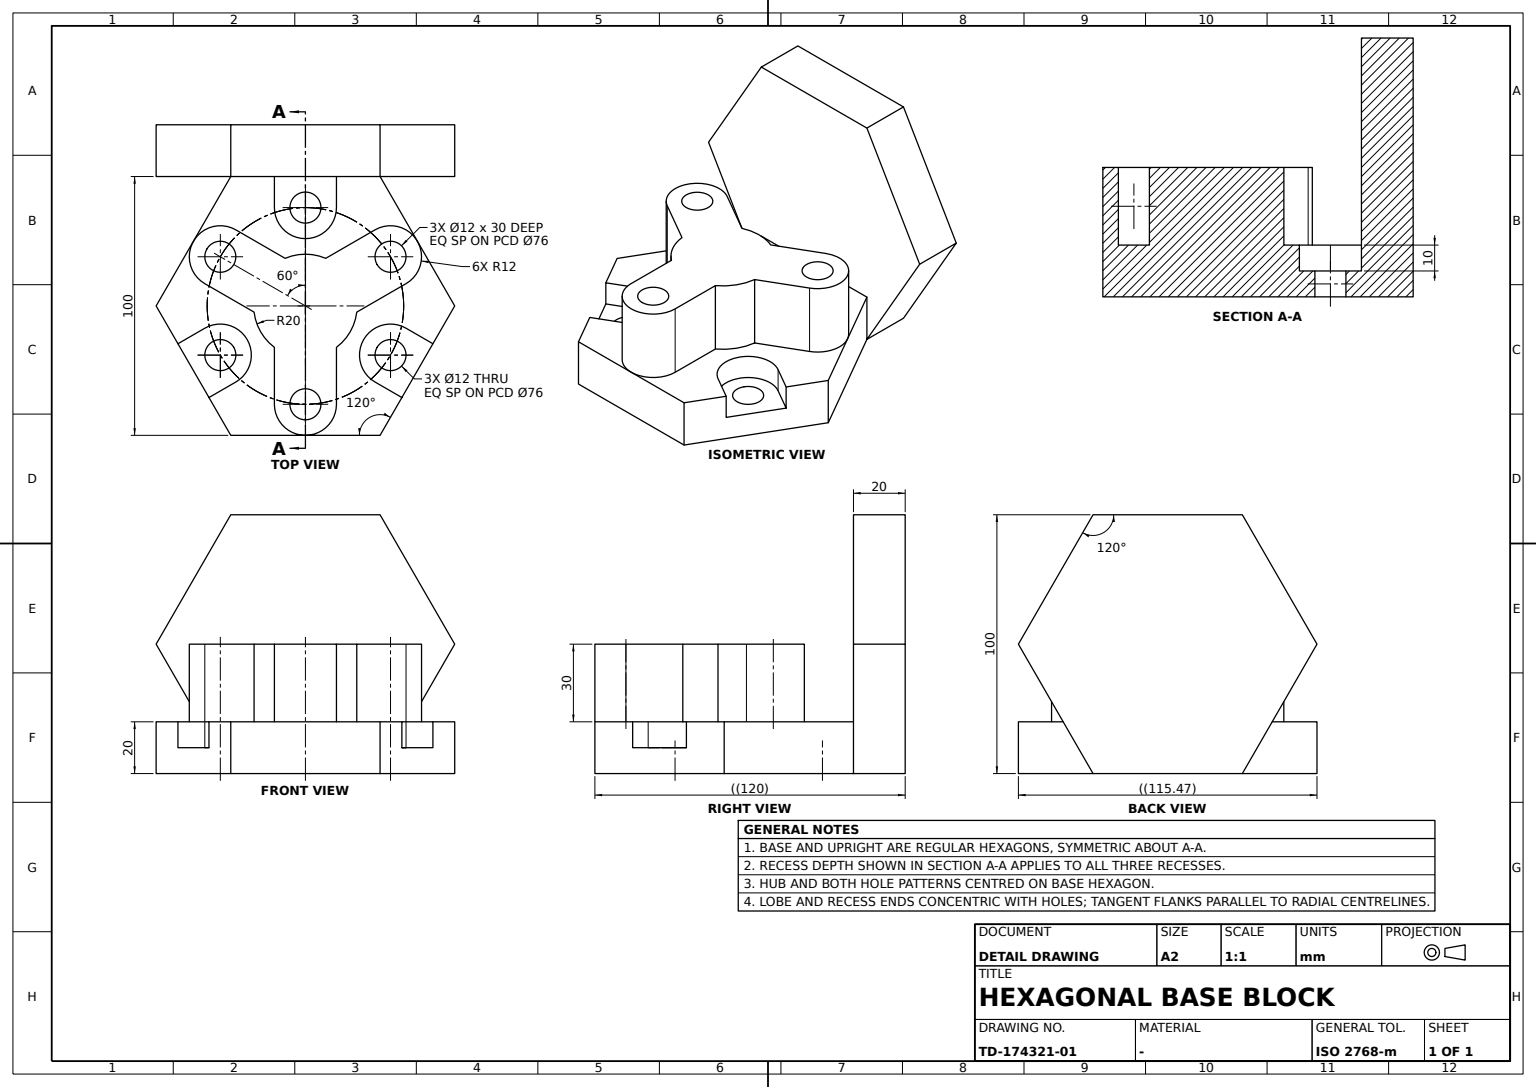
solid
v1 (-22,38.105118,20)
v2 (-22,38.105118,50)
e1 v1 v2 LINE
v3 (-13,32.908965,20)
e2 v3 v1 CIRCLE(AX(P(-19,32.908965,20),D(0,0,1),D(1,0,0)),6)
v4 (-13,32.908965,50)
e3 v4 v3 LINE
e4 v4 v2 CIRCLE(AX(P(-19,32.908965,50),D(0,0,1),D(1,0,0)),6)
face CYL(AX(P(-19,32.908965,35),D(0,0,-1),D(1,0,0)),6) rev [-e1 -e2 -e3 e4]
v5 (13.876084,29.787189,10)
v6 (16,27.712813,10)
e5 v5 v6 CIRCLE(AX(P(19,32.908965,10),D(0,0,1),D(1,0,0)),6)
v7 (24.123916,36.030741,10)
e6 v7 v5 CIRCLE(AX(P(19,32.908965,10),D(0,0,1),D(1,0,0)),6)
e7 v6 v7 CIRCLE(AX(P(19,32.908965,10),D(0,0,1),D(1,0,0)),6)
v8 (35.392305,37.30127,10)
v9 (14.607695,49.30127,10)
e8 v8 v9 LINE
v10 (8.607695,38.908965,10)
e9 v9 v10 LINE
v11 (13,22.51666,10)
e10 v10 v11 CIRCLE(AX(P(19,32.908965,10),D(0,0,1),D(-0.5,-0.866025404,0)),12)
v12 (29.392305,26.908965,10)
e11 v11 v12 CIRCLE(AX(P(19,32.908965,10),D(0,0,1),D(-0.5,-0.866025404,0)),12)
e12 v12 v8 LINE
face PLANE(AX(P(0,0,10),D(0,0,1),D(1,0,0))) [-e5 -e6 -e7] [e8 e9 e10 e11 e12]
v13 (-18.392305,7.856406,20)
v14 (-29.392305,26.908965,20)
e13 v13 v14 LINE
v15 (-18.392305,7.856406,50)
e14 v13 v15 LINE
v16 (-29.392305,26.908965,50)
e15 v15 v16 LINE
e16 v14 v16 LINE
face PLANE(AX(P(8.607695,-38.908965,20),D(0.866025404,0.5,0),D(0.5,-0.866025404,0))) rev [-e13 e14 e15 -e16]
v17 (-16,-27.712813,20)
v18 (-22,-38.105118,20)
e17 v17 v18 CIRCLE(AX(P(-19,-32.908965,20),D(0,0,1),D(1,0,0)),6)
v19 (-13,-32.908965,20)
e18 v18 v19 CIRCLE(AX(P(-19,-32.908965,20),D(0,0,1),D(1,0,0)),6)
e19 v19 v17 CIRCLE(AX(P(-19,-32.908965,20),D(0,0,1),D(1,0,0)),6)
face PLANE(AX(P(0,0,20),D(0,0,1),D(1,0,0))) [e17 e18 e19]
v20 (-25,-43.30127,20)
v21 (-29.392305,-26.908965,20)
e20 v20 v21 CIRCLE(AX(P(-19,-32.908965,20),D(0,0,-1),D(1,0,0)),12)
v22 (-18.392305,-7.856406,20)
e21 v21 v22 LINE
e22 v22 v13 CIRCLE(AX(P(0,0,20),D(0,0,-1),D(1,0,0)),20)
v23 (-25,43.30127,20)
e23 v14 v23 CIRCLE(AX(P(-19,32.908965,20),D(0,0,-1),D(1,0,0)),12)
v24 (-50,28.867513,20)
e24 v23 v24 LINE
v25 (-50,12,20)
e25 v24 v25 LINE
v26 (-38,12,20)
e26 v26 v25 LINE
v27 (-26,0,20)
e27 v27 v26 CIRCLE(AX(P(-38,0,20),D(0,0,1),D(1,0,0)),12)
v28 (-38,-12,20)
e28 v28 v27 CIRCLE(AX(P(-38,0,20),D(0,0,1),D(1,0,0)),12)
v29 (-50,-12,20)
e29 v29 v28 LINE
v30 (-50,-28.867513,20)
e30 v29 v30 LINE
e31 v30 v20 LINE
face PLANE(AX(P(0,0,20),D(0,0,1),D(1,0,0))) [e20 e21 e22 e13 e23 e24 e25 -e26 -e27 -e28 -e29 e30 e31]
v31 (13,-22.51666,20)
v32 (8.607695,-38.908965,20)
e32 v31 v32 CIRCLE(AX(P(19,-32.908965,20),D(0,0,1),D(-0.5,0.866025404,0)),12)
v33 (29.392305,-26.908965,20)
e33 v33 v31 CIRCLE(AX(P(19,-32.908965,20),D(0,0,1),D(-0.5,0.866025404,0)),12)
v34 (35.392305,-37.30127,20)
e34 v34 v33 LINE
v35 (50,-28.867513,20)
e35 v34 v35 LINE
v36 (50,0,20)
e36 v35 v36 LINE
v37 (38,-12,20)
e37 v36 v37 CIRCLE(AX(P(38,0,20),D(0,0,-1),D(1,0,0)),12)
v38 (16,-12,20)
e38 v37 v38 LINE
v39 (2.392305,-19.856406,20)
e39 v38 v39 CIRCLE(AX(P(0,0,20),D(0,0,-1),D(1,0,0)),20)
v40 (-8.607695,-38.908965,20)
e40 v39 v40 LINE
e41 v40 v20 CIRCLE(AX(P(-19,-32.908965,20),D(0,0,-1),D(1,0,0)),12)
v41 (0,-57.735027,20)
e42 v20 v41 LINE
v42 (14.607695,-49.30127,20)
e43 v41 v42 LINE
e44 v32 v42 LINE
face PLANE(AX(P(0,0,20),D(0,0,1),D(1,0,0))) [-e32 -e33 -e34 e35 e36 e37 e38 e39 e40 e41 e42 e43 -e44]
v43 (-70,-57.735027,50)
v44 (-70,-28.867513,100)
e45 v43 v44 LINE
v45 (-50,-57.735027,50)
e46 v45 v43 LINE
v46 (-50,-28.867513,100)
e47 v45 v46 LINE
e48 v46 v44 LINE
face PLANE(AX(P(-50,-57.735027,50),D(0,-0.866025404,0.5),D(0,0.5,0.866025404))) [-e45 -e46 e47 e48]
v47 (2.392305,19.856406,50)
v48 (16,12,50)
e49 v47 v48 CIRCLE(AX(P(0,0,50),D(0,0,-1),D(1,0,0)),20)
v49 (16,12,20)
e50 v49 v48 LINE
v50 (2.392305,19.856406,20)
e51 v50 v49 CIRCLE(AX(P(0,0,20),D(0,0,-1),D(1,0,0)),20)
e52 v50 v47 LINE
face CYL(AX(P(0,0,35),D(0,0,-1),D(1,0,0)),20) [e49 -e50 -e51 e52]
v51 (16,-27.712813,10)
v52 (19.14158,-38.907295,10)
e53 v51 v52 CIRCLE(AX(P(19,-32.908965,10),D(0,0,1),D(1,0,0)),6)
v53 (18.85842,-26.910636,10)
e54 v53 v51 CIRCLE(AX(P(19,-32.908965,10),D(0,0,1),D(1,0,0)),6)
e55 v52 v53 CIRCLE(AX(P(19,-32.908965,10),D(0,0,1),D(1,0,0)),6)
v54 (35.392305,-37.30127,10)
v55 (29.392305,-26.908965,10)
e56 v54 v55 LINE
v56 (13,-22.51666,10)
e57 v55 v56 CIRCLE(AX(P(19,-32.908965,10),D(0,0,1),D(-0.5,0.866025404,0)),12)
v57 (8.607695,-38.908965,10)
e58 v56 v57 CIRCLE(AX(P(19,-32.908965,10),D(0,0,1),D(-0.5,0.866025404,0)),12)
v58 (14.607695,-49.30127,10)
e59 v57 v58 LINE
e60 v58 v54 LINE
face PLANE(AX(P(0,0,10),D(0,0,1),D(1,0,0))) [-e53 -e54 -e55] [e56 e57 e58 e59 e60]
v59 (-50,-12,10)
e61 v29 v59 LINE
v60 (-50,12,10)
e62 v60 v59 LINE
e63 v25 v60 LINE
v61 (-50,28.867513,0)
e64 v61 v24 LINE
v62 (-50,57.735027,50)
e65 v62 v61 LINE
v63 (-50,28.867513,100)
e66 v63 v62 LINE
e67 v46 v63 LINE
v64 (-50,-28.867513,0)
e68 v64 v45 LINE
e69 v64 v30 LINE
face PLANE(AX(P(-50,28.867513,0),D(-1,0,0),D(0,-1,0))) rev [-e30 e61 -e62 -e63 -e25 -e64 -e65 -e66 -e67 -e47 -e68 e69]
v65 (-32,0,0)
v66 (-32,0,10)
e70 v65 v66 LINE
v67 (-43.265495,2.876553,10)
e71 v66 v67 CIRCLE(AX(P(-38,0,10),D(0,0,1),D(1,0,0)),6)
v68 (-43.265495,2.876553,0)
e72 v68 v67 LINE
e73 v68 v65 CIRCLE(AX(P(-38,0,0),D(0,0,-1),D(1,0,0)),6)
face CYL(AX(P(-38,0,9.9),D(0,0,1),D(1,0,0)),6) rev [e70 e71 -e72 e73]
e74 v42 v58 LINE
e75 v32 v57 LINE
face PLANE(AX(P(8.607695,-38.908965,20),D(0.866025404,0.5,0),D(0.5,-0.866025404,0))) [e74 -e59 -e75 e44]
v69 (-22,-38.105118,50)
e76 v18 v69 LINE
v70 (-16,-27.712813,50)
e77 v17 v70 LINE
e78 v70 v69 CIRCLE(AX(P(-19,-32.908965,50),D(0,0,1),D(1,0,0)),6)
face CYL(AX(P(-19,-32.908965,35),D(0,0,-1),D(1,0,0)),6) rev [-e76 -e17 e77 e78]
v71 (-32.734505,-2.876553,10)
e79 v67 v71 CIRCLE(AX(P(-38,0,10),D(0,0,1),D(1,0,0)),6)
e80 v71 v66 CIRCLE(AX(P(-38,0,10),D(0,0,1),D(1,0,0)),6)
v72 (-38,-12,10)
e81 v59 v72 LINE
v73 (-26,0,10)
e82 v72 v73 CIRCLE(AX(P(-38,0,10),D(0,0,1),D(1,0,0)),12)
v74 (-38,12,10)
e83 v73 v74 CIRCLE(AX(P(-38,0,10),D(0,0,1),D(1,0,0)),12)
e84 v74 v60 LINE
face PLANE(AX(P(0,0,10),D(0,0,1),D(1,0,0))) [-e79 -e71 -e80] [e62 e81 e82 e83 e84]
v75 (-16,27.712813,20)
v76 (-16,27.712813,50)
e85 v75 v76 LINE
e86 v1 v75 CIRCLE(AX(P(-19,32.908965,20),D(0,0,1),D(1,0,0)),6)
e87 v2 v76 CIRCLE(AX(P(-19,32.908965,50),D(0,0,1),D(1,0,0)),6)
face CYL(AX(P(-19,32.908965,35),D(0,0,-1),D(1,0,0)),6) rev [-e85 -e86 e1 e87]
v77 (19.14158,-38.907295,0)
e88 v77 v52 LINE
v78 (16,-27.712813,0)
e89 v77 v78 CIRCLE(AX(P(19,-32.908965,0),D(0,0,-1),D(-0.5,0.866025404,0)),6)
e90 v78 v51 LINE
face CYL(AX(P(19,-32.908965,9.9),D(0,0,1),D(-0.5,0.866025404,0)),6) rev [e53 -e88 e89 e90]
v79 (50,28.867513,20)
e91 v36 v79 LINE
v80 (35.392305,37.30127,20)
e92 v79 v80 LINE
v81 (29.392305,26.908965,20)
e93 v81 v80 LINE
v82 (13,22.51666,20)
e94 v82 v81 CIRCLE(AX(P(19,32.908965,20),D(0,0,1),D(-0.5,-0.866025404,0)),12)
v83 (8.607695,38.908965,20)
e95 v83 v82 CIRCLE(AX(P(19,32.908965,20),D(0,0,1),D(-0.5,-0.866025404,0)),12)
v84 (14.607695,49.30127,20)
e96 v84 v83 LINE
v85 (0,57.735027,20)
e97 v84 v85 LINE
e98 v85 v23 LINE
v86 (-8.607695,38.908965,20)
e99 v23 v86 CIRCLE(AX(P(-19,32.908965,20),D(0,0,-1),D(1,0,0)),12)
e100 v86 v50 LINE
v87 (38,12,20)
e101 v49 v87 LINE
e102 v87 v36 CIRCLE(AX(P(38,0,20),D(0,0,-1),D(1,0,0)),12)
face PLANE(AX(P(0,0,20),D(0,0,1),D(1,0,0))) [e91 e92 -e93 -e94 -e95 -e96 e97 e98 e99 e100 e51 e101 e102]
v88 (-70,28.867513,0)
e103 v61 v88 LINE
v89 (-70,57.735027,50)
e104 v89 v88 LINE
e105 v62 v89 LINE
face PLANE(AX(P(-50,57.735027,50),D(0,0.866025404,-0.5),D(0,-0.5,-0.866025404))) [e103 -e104 -e105 e65]
e106 v83 v10 LINE
e107 v82 v11 LINE
face CYL(AX(P(19,32.908965,15),D(0,0,-1),D(-0.5,-0.866025404,0)),12) rev [-e10 -e106 e95 e107]
v90 (38,12,50)
e108 v87 v90 LINE
e109 v48 v90 LINE
face PLANE(AX(P(-38,12,20),D(0,-1,0),D(-1,0,0))) rev [-e108 -e101 e50 e109]
e110 v33 v55 LINE
e111 v34 v54 LINE
face PLANE(AX(P(29.392305,-26.908965,20),D(0.866025404,0.5,0),D(0.5,-0.866025404,0))) rev [e110 -e56 -e111 e34]
e112 v28 v72 LINE
e113 v27 v73 LINE
face CYL(AX(P(-38,0,15),D(0,0,-1),D(1,0,0)),12) rev [-e112 e28 e113 -e82]
e114 v84 v9 LINE
face PLANE(AX(P(8.607695,38.908965,20),D(-0.866025404,0.5,0),D(0.5,0.866025404,0))) rev [-e114 e96 e106 -e9]
e115 v31 v56 LINE
face CYL(AX(P(19,-32.908965,15),D(0,0,-1),D(-0.5,0.866025404,0)),12) rev [-e57 -e110 e33 e115]
face PLANE(AX(P(-38,-12,20),D(0,-1,0),D(-1,0,0))) rev [-e81 -e61 e29 e112]
e116 v81 v12 LINE
e117 v80 v8 LINE
face PLANE(AX(P(29.392305,26.908965,20),D(-0.866025404,0.5,0),D(0.5,0.866025404,0))) [-e116 e93 e117 -e12]
v91 (16,-12,50)
e118 v38 v91 LINE
v92 (38,-12,50)
e119 v37 v92 LINE
e120 v92 v91 LINE
face PLANE(AX(P(-38,-12,20),D(0,-1,0),D(-1,0,0))) [-e118 -e38 e119 e120]
v93 (18.85842,-26.910636,0)
e121 v78 v93 CIRCLE(AX(P(19,-32.908965,0),D(0,0,-1),D(-0.5,0.866025404,0)),6)
e122 v93 v77 CIRCLE(AX(P(19,-32.908965,0),D(0,0,-1),D(-0.5,0.866025404,0)),6)
v94 (0,57.735027,0)
e123 v94 v61 LINE
v95 (50,28.867513,0)
e124 v95 v94 LINE
v96 (50,-28.867513,0)
e125 v96 v95 LINE
v97 (0,-57.735027,0)
e126 v97 v96 LINE
e127 v64 v97 LINE
v98 (-70,-28.867513,0)
e128 v64 v98 LINE
e129 v88 v98 LINE
v99 (-32.734505,-2.876553,0)
e130 v99 v68 CIRCLE(AX(P(-38,0,0),D(0,0,-1),D(1,0,0)),6)
e131 v65 v99 CIRCLE(AX(P(-38,0,0),D(0,0,-1),D(1,0,0)),6)
v100 (13.876084,29.787189,0)
v101 (24.123916,36.030741,0)
e132 v100 v101 CIRCLE(AX(P(19,32.908965,0),D(0,0,-1),D(-0.5,-0.866025404,0)),6)
v102 (16,27.712813,0)
e133 v102 v100 CIRCLE(AX(P(19,32.908965,0),D(0,0,-1),D(-0.5,-0.866025404,0)),6)
e134 v101 v102 CIRCLE(AX(P(19,32.908965,0),D(0,0,-1),D(-0.5,-0.866025404,0)),6)
face PLANE(AX(P(0,0,0),D(0,0,1),D(1,0,0))) rev [-e121 -e89 -e122] [-e123 -e124 -e125 -e126 -e127 e128 -e129 -e103] [-e73 -e130 -e131] [-e132 -e133 -e134]
e135 v93 v53 LINE
face CYL(AX(P(19,-32.908965,9.9),D(0,0,1),D(-0.5,0.866025404,0)),6) rev [e55 -e135 e122 e88]
v103 (32,0,20)
v104 (44,0,20)
e136 v103 v104 CIRCLE(AX(P(38,0,20),D(0,0,1),D(1,0,0)),6)
v105 (32,0,50)
e137 v103 v105 LINE
v106 (44,0,50)
e138 v105 v106 CIRCLE(AX(P(38,0,50),D(0,0,1),D(1,0,0)),6)
e139 v104 v106 LINE
face CYL(AX(P(38,0,35),D(0,0,-1),D(1,0,0)),6) rev [-e136 e137 e138 -e139]
v107 (-13,-32.908965,50)
e140 v107 v19 LINE
e141 v107 v70 CIRCLE(AX(P(-19,-32.908965,50),D(0,0,1),D(1,0,0)),6)
face CYL(AX(P(-19,-32.908965,35),D(0,0,-1),D(1,0,0)),6) rev [-e77 -e19 -e140 e141]
e142 v75 v3 CIRCLE(AX(P(-19,32.908965,20),D(0,0,1),D(1,0,0)),6)
face PLANE(AX(P(0,0,20),D(0,0,1),D(1,0,0))) [e142 e2 e86]
e143 v95 v79 LINE
e144 v96 v35 LINE
face PLANE(AX(P(50,-28.867513,0),D(1,0,0),D(0,1,0))) [e125 e143 -e91 -e36 -e144]
v108 (2.392305,-19.856406,50)
e145 v91 v108 CIRCLE(AX(P(0,0,50),D(0,0,-1),D(1,0,0)),20)
e146 v39 v108 LINE
face CYL(AX(P(0,0,35),D(0,0,-1),D(1,0,0)),20) [e145 -e146 -e39 e118]
e147 v100 v5 LINE
e148 v101 v7 LINE
face CYL(AX(P(19,32.908965,9.9),D(0,0,1),D(-0.5,-0.866025404,0)),6) rev [-e147 e132 e148 e6]
e149 v76 v4 CIRCLE(AX(P(-19,32.908965,50),D(0,0,1),D(1,0,0)),6)
face CYL(AX(P(-19,32.908965,35),D(0,0,-1),D(1,0,0)),6) rev [-e142 e85 e149 e3]
e150 v94 v85 LINE
face PLANE(AX(P(0,57.735027,0),D(-0.5,0.866025404,0),D(-0.866025404,-0.5,0))) [-e24 -e98 -e150 e123 e64]
e151 v104 v103 CIRCLE(AX(P(38,0,20),D(0,0,1),D(1,0,0)),6)
face PLANE(AX(P(0,0,20),D(0,0,1),D(1,0,0))) [e151 e136]
v109 (-8.607695,-38.908965,50)
e152 v108 v109 LINE
e153 v40 v109 LINE
face PLANE(AX(P(29.392305,26.908965,20),D(-0.866025404,0.5,0),D(0.5,0.866025404,0))) rev [e152 -e153 -e40 e146]
v110 (-29.392305,-26.908965,50)
e154 v109 v110 CIRCLE(AX(P(-19,-32.908965,50),D(0,0,-1),D(1,0,0)),12)
e155 v21 v110 LINE
face CYL(AX(P(-19,-32.908965,35),D(0,0,-1),D(1,0,0)),12) [-e20 -e41 e153 e154 -e155]
e156 v26 v74 LINE
face PLANE(AX(P(-38,12,20),D(0,-1,0),D(-1,0,0))) [e63 -e84 -e156 e26]
e157 v102 v6 LINE
face CYL(AX(P(19,32.908965,9.9),D(0,0,1),D(-0.5,-0.866025404,0)),6) rev [e7 -e148 e134 e157]
face PLANE(AX(P(50,28.867513,0),D(0.5,0.866025404,0),D(-0.866025404,0.5,0))) [-e92 -e143 e124 e150 -e97 e114 -e8 -e117]
v111 (50,0,50)
e158 v111 v92 CIRCLE(AX(P(38,0,50),D(0,0,-1),D(1,0,0)),12)
e159 v111 v36 LINE
face CYL(AX(P(38,0,35),D(0,0,-1),D(1,0,0)),12) [e158 -e119 -e37 -e159]
e160 v106 v105 CIRCLE(AX(P(38,0,50),D(0,0,1),D(1,0,0)),6)
face CYL(AX(P(38,0,35),D(0,0,-1),D(1,0,0)),6) rev [e160 -e137 -e151 e139]
e161 v97 v41 LINE
face PLANE(AX(P(-50,-28.867513,0),D(-0.5,-0.866025404,0),D(0.866025404,-0.5,0))) [-e31 -e69 e127 e161 -e42]
e162 v99 v71 LINE
face CYL(AX(P(-38,0,9.9),D(0,0,1),D(1,0,0)),6) rev [e131 e162 e80 -e70]
face CYL(AX(P(19,32.908965,15),D(0,0,-1),D(-0.5,-0.866025404,0)),12) rev [-e11 -e107 e94 e116]
e163 v90 v111 CIRCLE(AX(P(38,0,50),D(0,0,-1),D(1,0,0)),12)
face CYL(AX(P(38,0,35),D(0,0,-1),D(1,0,0)),12) [e159 -e102 e108 e163]
face CYL(AX(P(-38,0,15),D(0,0,-1),D(1,0,0)),12) rev [e156 -e83 -e113 e27]
e164 v98 v43 LINE
face PLANE(AX(P(-50,-28.867513,0),D(0,-0.866025404,-0.5),D(0,-0.5,0.866025404))) [-e164 -e128 e68 e46]
face CYL(AX(P(19,-32.908965,9.9),D(0,0,1),D(-0.5,0.866025404,0)),6) rev [e54 -e90 e121 e135]
e165 v69 v107 CIRCLE(AX(P(-19,-32.908965,50),D(0,0,1),D(1,0,0)),6)
v112 (-8.607695,38.908965,50)
e166 v112 v47 LINE
e167 v16 v112 CIRCLE(AX(P(-19,32.908965,50),D(0,0,-1),D(1,0,0)),12)
v113 (-18.392305,-7.856406,50)
e168 v113 v15 CIRCLE(AX(P(0,0,50),D(0,0,-1),D(1,0,0)),20)
e169 v110 v113 LINE
face PLANE(AX(P(0,0,50),D(0,0,1),D(1,0,0))) [-e160 -e138] [-e149 -e87 -e4] [-e141 -e165 -e78] [-e120 -e158 -e163 -e109 -e49 -e166 -e167 -e15 -e168 -e169 -e154 -e152 -e145]
face PLANE(AX(P(0,-57.735027,0),D(0.5,-0.866025404,0),D(0.866025404,0.5,0))) [-e43 -e161 e126 e144 -e35 e111 -e60 -e74]
e170 v86 v112 LINE
face CYL(AX(P(-19,32.908965,35),D(0,0,-1),D(1,0,0)),12) [-e170 -e99 -e23 e16 e167]
v114 (-70,28.867513,100)
e171 v114 v89 LINE
e172 v44 v114 LINE
face PLANE(AX(P(-70,0,50),D(-1,0,0),D(0,0,1))) [e171 e104 e129 e164 e45 e172]
face PLANE(AX(P(29.392305,-26.908965,20),D(0.866025404,0.5,0),D(0.5,-0.866025404,0))) [-e52 -e100 e170 e166]
e173 v63 v114 LINE
face PLANE(AX(P(-50,28.867513,100),D(0,0.866025404,0.5),D(0,0.5,-0.866025404))) [-e173 e66 e105 -e171]
face PLANE(AX(P(-50,-28.867513,100),D(0,0,1),D(0,1,0))) [-e48 e67 e173 -e172]
face CYL(AX(P(-38,0,9.9),D(0,0,1),D(1,0,0)),6) rev [e72 e79 -e162 e130]
face CYL(AX(P(19,-32.908965,15),D(0,0,-1),D(-0.5,0.866025404,0)),12) rev [-e58 -e115 e32 e75]
e174 v22 v113 LINE
face PLANE(AX(P(8.607695,38.908965,20),D(-0.866025404,0.5,0),D(0.5,0.866025404,0))) [e155 e169 -e174 -e21]
face CYL(AX(P(-19,-32.908965,35),D(0,0,-1),D(1,0,0)),6) rev [e76 e165 e140 -e18]
face CYL(AX(P(0,0,35),D(0,0,-1),D(1,0,0)),20) [e168 -e14 -e22 e174]
face CYL(AX(P(19,32.908965,9.9),D(0,0,1),D(-0.5,-0.866025404,0)),6) rev [-e157 e133 e147 e5]
